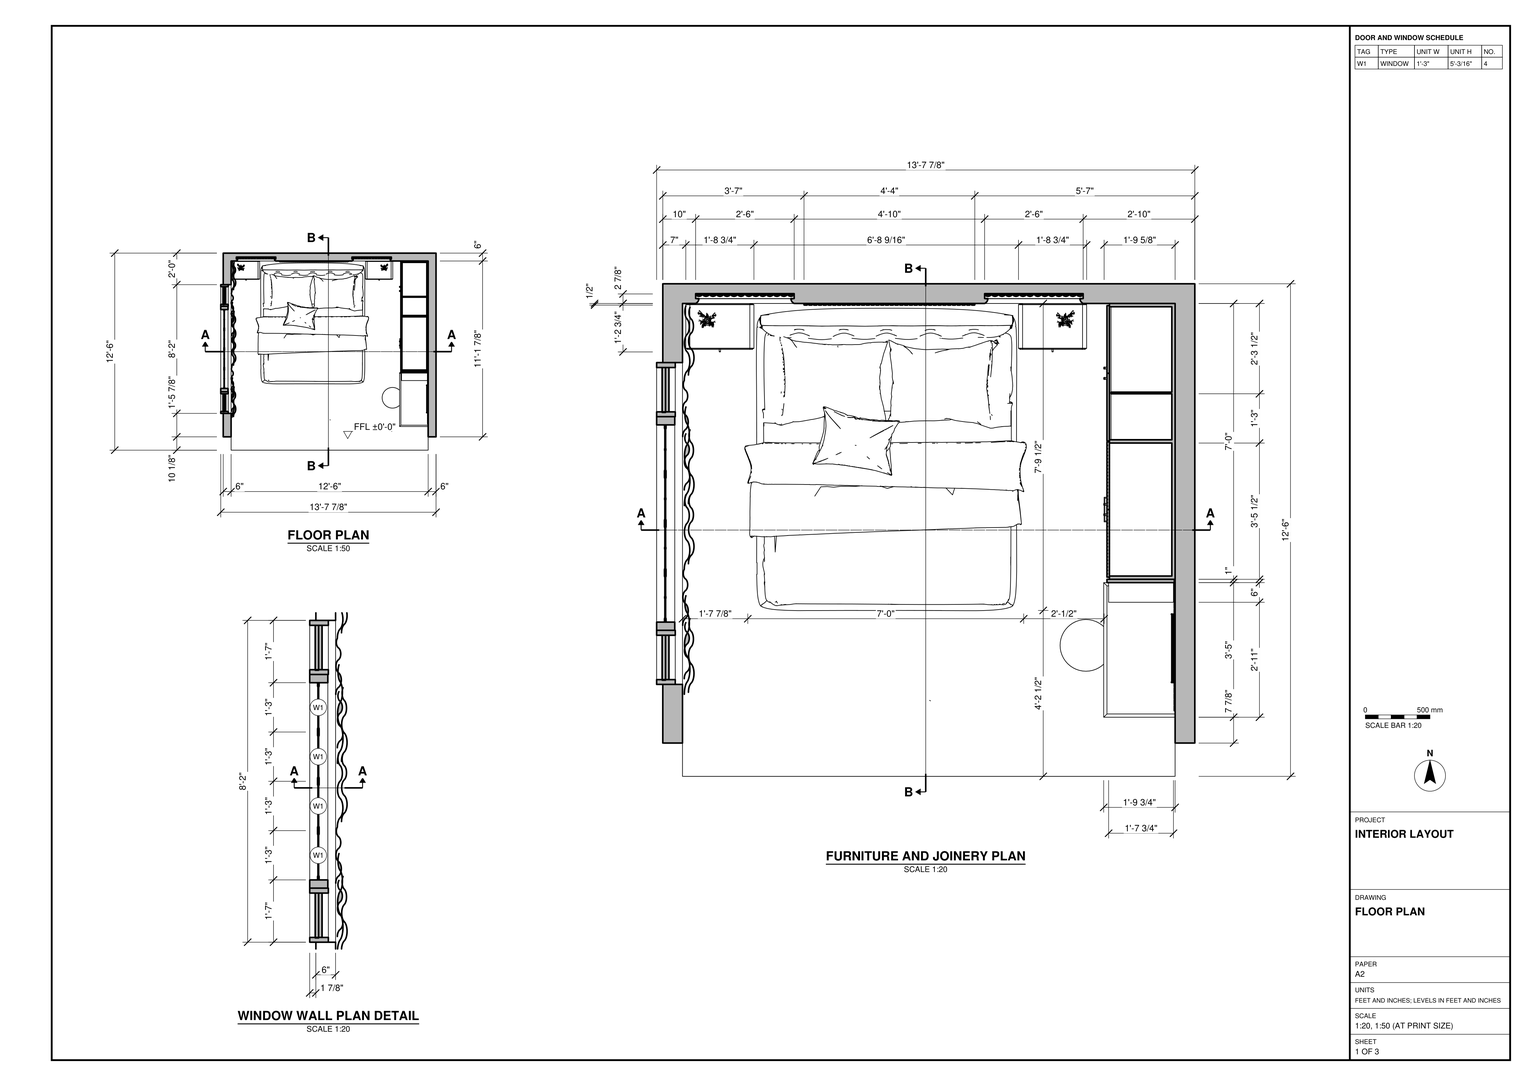
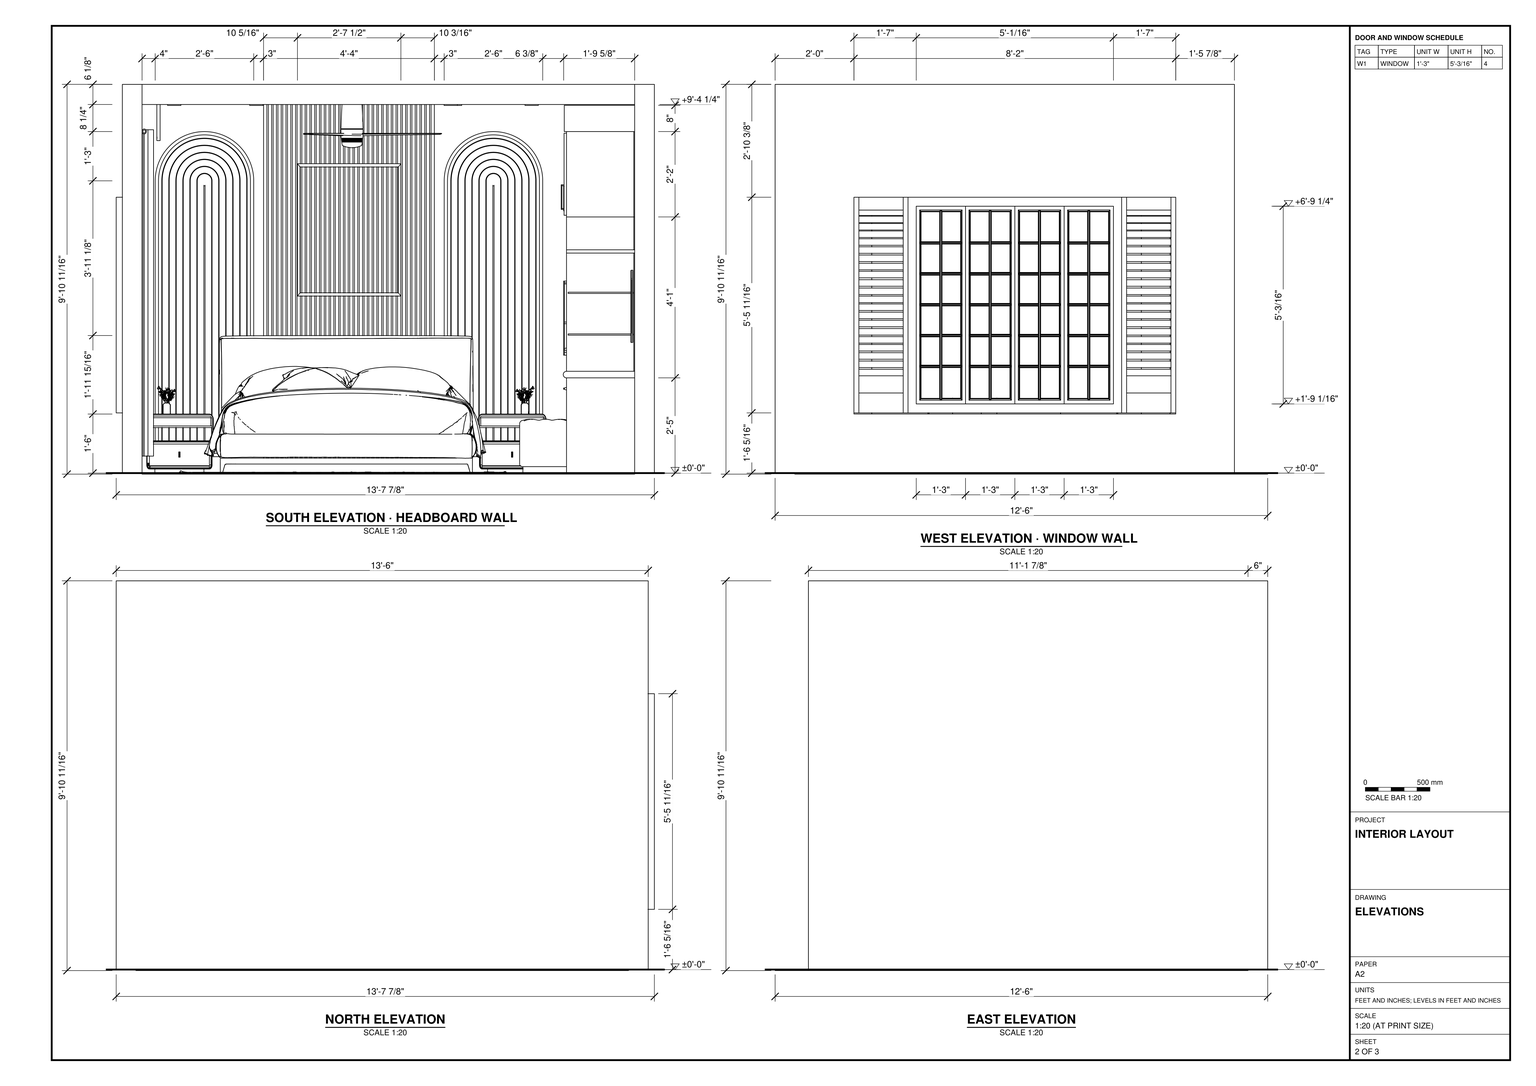
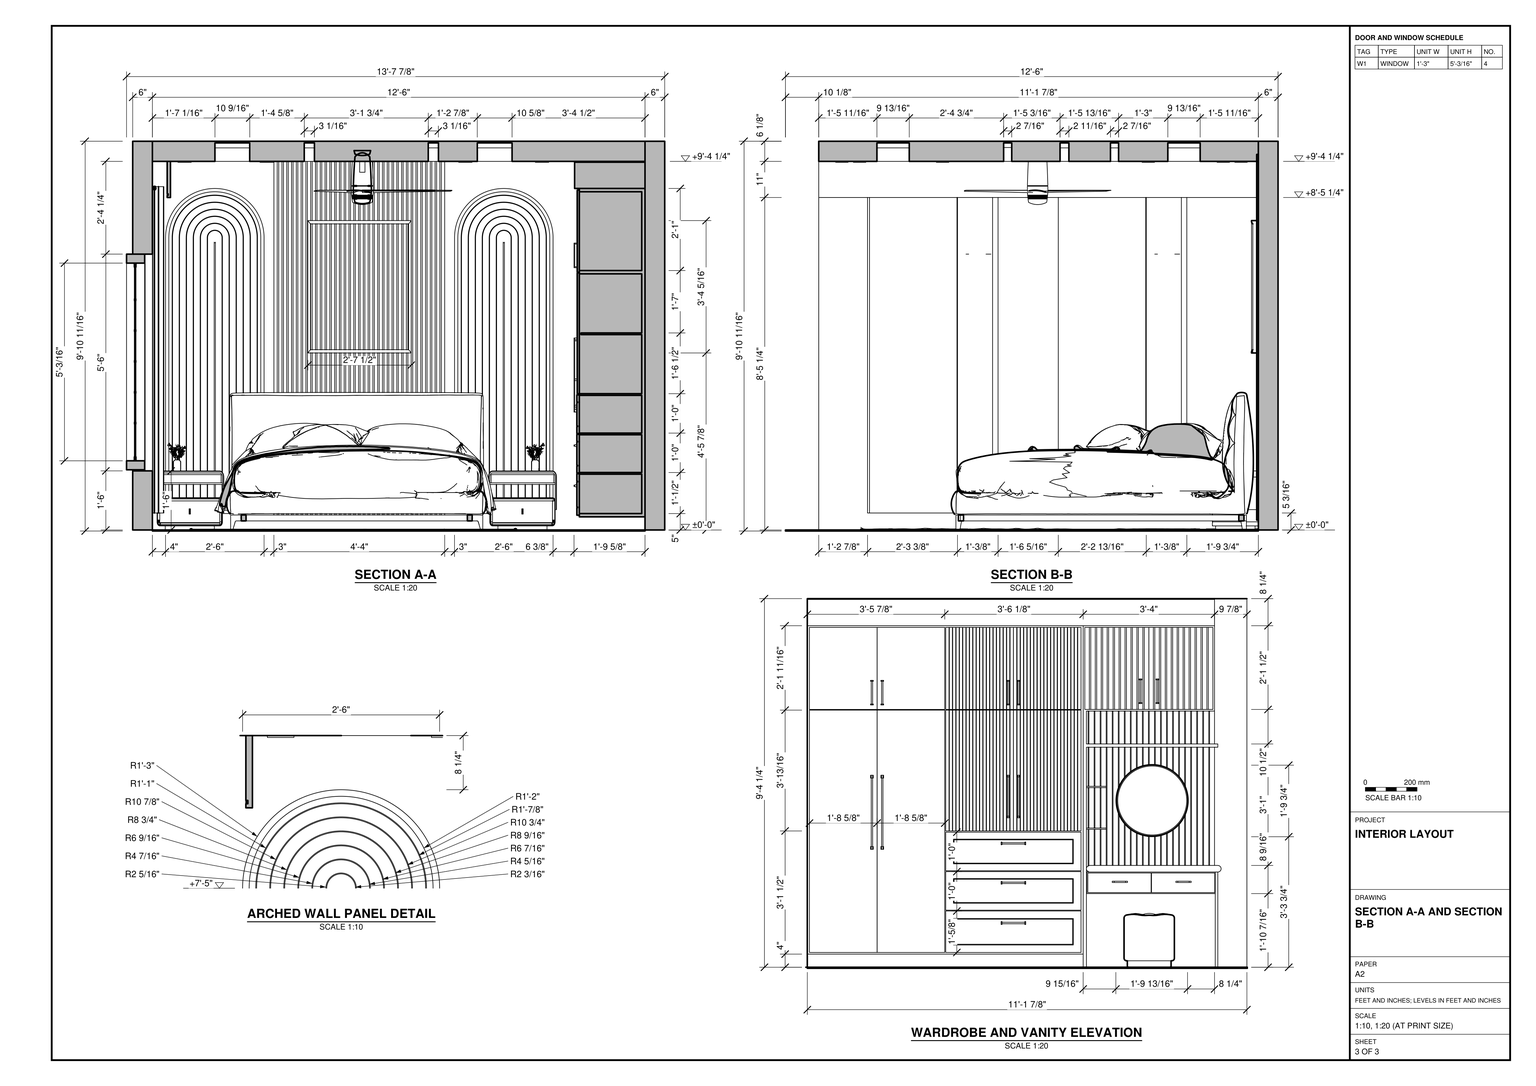
Build the furnished bedroom in SketchUp using task_files/diagram_01.pdf. Work in feet and inches. Set the finished floor at ±0'-0". The overall model is 13'-7 7/8" wide, 12'-6" deep and 9'-10 11/16" high. Model the floor, the 6" walls and the ceiling shown in section, leaving the side opposite the headboard open as drawn in plan.

Use the window wall detail to place the four glazed window units in a single framed opening, with the horizontally slatted panels at its ends and curtains on the room side. Set the bed against the headboard wall with a low bedside unit on each side. Follow the arched panel detail for the nested bands above the bedside units and the elevation for the vertically ribbed panel behind the bed. Include the framed art above the headboard and the ceiling fan over the bed.

Fit the wardrobe and vanity along the wall opposite the windows. Use the joinery elevation to distinguish the tall doors, the ribbed doors above the drawer bank, and the vanity bay with its overhead cupboard, round mirror, work surface and seat. Decor and loose items may be any suitable library components. Keep shell elements and each furniture or joinery piece in separate groups or components, and use components for repeated parts. Save one SketchUp model as output_files/bedroom_with_arched_headboard_wall_and_fitted_wardrobes.skp.

# SketchUp Ruby script. Lengths in inches.
U = 1.inch
M = Sketchup.active_model
def pt(a) = Geom::Point3d.new(a.map { |v| v * U })
def face(e, loops, mat)
  f = e.add_face(loops[0].map { |a| pt(a) })
  loops[1..].each { |l| e.add_face(l.map { |a| pt(a) }).erase! }
  f.material = f.back_material = mat if mat
  f
end
# faces: each face lists its corners as indices into pts; further lists are holes
def faces(e, pts, list, mat = nil) = list.each { |f| face(e, (f[0].is_a?(Array) ? f : [f]).map { |l| l.map { |i| pts[i] } }, mat) }
# xy, xz, yz: faces in a plane at the given z, y or x. An outline is a flat list of corners, or four numbers for a rectangle; further outlines are holes
def ring(l) = l.size == 4 ? [[l[0], l[1]], [l[2], l[1]], [l[2], l[3]], [l[0], l[3]]] : l.each_slice(2).to_a
def flat(e, list, mat, &to3) = list.each { |f| face(e, (f[0].is_a?(Array) ? f : [f]).map { |l| ring(l).map { |u, v| to3.(u, v) } }, mat) }
def xy(e, z, list, mat = nil) = flat(e, list, mat) { |x, y| [x, y, z] }
def xz(e, y, list, mat = nil) = flat(e, list, mat) { |x, z| [x, y, z] }
def yz(e, x, list, mat = nil) = flat(e, list, mat) { |y, z| [x, y, z] }
def lines(e, pts, list) = list.each { |a, b| e.add_line(pt(pts[a]), pt(pts[b])) }
# prism: a flat outline (further loops are holes) pulled along v
def prism(e, loops, v, mat = nil)
  f = face(e, loops, mat); d = Geom::Vector3d.new(v.map { |x| x * U })
  f.pushpull(f.normal.samedirection?(d) ? d.length : -d.length)
end
def box(e, o, s, mat = nil) = prism(e, [[o, [o[0] + s[0], o[1], o[2]], [o[0] + s[0], o[1] + s[1], o[2]], [o[0], o[1] + s[1], o[2]]]], [0, 0, s[2]], mat)
def at(x, y, z, deg = 0) = Geom::Transformation.translation(pt([x, y, z])) * Geom::Transformation.rotation(ORIGIN, Z_AXIS, deg.degrees)
def axes(o, x, y, z) = Geom::Transformation.new([*x, 0, *y, 0, *z, 0, *pt(o).to_a, 1])
def part(name) = M.definitions.add(name)
# library, detail: a bought-in or finely detailed component or shape, given as its bounding box
def library(name, o, s) = part(name).tap { |d| box(d.entities, o, s) }
def detail(e, o, s) = box(e.add_group.entities, o, s)
def put(e, d, t, mat = nil) = e.add_instance(d, t).tap { |i| i.material = mat if mat }
def group(e, t, mat = nil) = e.add_group.tap { |g| g.transformation = t; g.material = mat if mat }.entities
root = M.entities
M.materials.add("Carpet_Frieze_Low").color = [170, 156, 146]
M.materials.add("Carpet_Loop_Low").color = [201, 172, 127]
M.materials["Carpet_Loop_Low"].alpha = 0.3
M.materials.add("[Marble Carrara Gold Floor Tile]").color = [225, 223, 217]
c1 = part("Curtain panel")
p = [[17.625,0.0625,78.74],[17.625,0.0625,0],[18.27,0,0],[18.27,0,78.74],[18.92,0.0625,0],[18.92,0.0625,78.74],
  [17,0.25,78.74],[17,0.25,0],[19.55,0.25,0],[19.55,0.25,78.74],[16.43,0.56,78.74],[16.43,0.56,0],
  [20.12,0.56,0],[20.12,0.56,78.74],[6.31,0.6,78.74],[6.31,0.6,0],[6.8125,0.45,0],[6.8125,0.45,78.74],
  [7.33,0.4,0],[7.33,0.4,78.74],[7.86,0.45,0],[7.86,0.45,78.74],[8.36,0.6,0],[8.36,0.6,78.74],
  [5.85,0.85,78.74],[5.85,0.85,0],[8.82,0.85,0],[8.82,0.85,78.74],[15.92,0.97,78.74],[15.92,0.97,0],
  [20.625,0.97,0],[20.625,0.97,78.74],[5.44,1.18,78.74],[5.44,1.18,0],[9.23,1.18,0],[9.23,1.18,78.74],
  [15.51,1.48,78.74],[15.51,1.48,0],[21.04,1.48,0],[21.04,1.48,78.74],[5.11,1.59,78.74],[5.11,1.59,0],
  [9.5625,1.59,0],[9.5625,1.59,78.74],[14.93,2.55,78.74],[14.93,2.55,0],[15.2,2.04,0],[15.2,2.04,78.74],
  [21.34,2.04,0],[21.64,2.59,0],[21.64,2.59,78.74],[21.34,2.04,78.74],[4.63,2.47,78.74],[4.63,2.47,0],
  [4.86,2.04,0],[4.86,2.04,78.74],[9.81,2.04,0],[10.08,2.55,0],[10.08,2.55,78.74],[9.81,2.04,78.74],
  [4.32,2.85,78.74],[4.32,2.85,0],[10.44,2.99,0],[10.44,2.99,78.74],[14.57,2.99,78.74],[14.57,2.99,0],
  [22.03,3.0625,0],[22.03,3.0625,78.74],[0.85,2.85,78.74],[0.85,2.85,0],[1.22,3.15,0],[1.22,3.15,78.74],
  [3.95,3.15,78.74],[3.95,3.15,0],[10.89,3.35,0],[10.89,3.35,78.74],[14.125,3.35,78.74],[14.125,3.35,0],
  [22.5,3.45,0],[22.5,3.45,78.74],[1.65,3.375,0],[1.65,3.375,78.74],[3.53,3.375,78.74],[3.53,3.375,0],
  [2.11,3.52,0],[2.11,3.52,78.74],[3.07,3.52,78.74],[3.07,3.52,0],[11.39,3.625,0],[11.39,3.625,78.74],
  [13.62,3.625,78.74],[13.62,3.625,0],[2.59,3.5625,0],[2.59,3.5625,78.74],[23.04,3.74,0],[23.04,3.74,78.74],
  [11.9375,3.79,0],[11.9375,3.79,78.74],[13.07,3.79,78.74],[13.07,3.79,0],[23.63,3.92,0],[23.63,3.92,78.74],
  [12.51,3.85,0],[12.51,3.85,78.74],[24.25,3.98,0],[24.25,3.98,78.74],[5.51,1.25,0],[5.9,0.93,0],
  [4.95,2.09,0],[5.1875,1.64,0],[6.35,0.69,0],[6.83,0.55,0],[7.33,0.5,0],[7.84,0.55,0],
  [8.32,0.69,0],[8.77,0.93,0],[9.16,1.25,0],[9.48,1.64,0],[9.72,2.09,0],[10,2.61,0],
  [10.375,3.0625,0],[10.83,3.4375,0],[17.64,0.16,0],[18.27,0.1,0],[11.35,3.71,0],[11.92,3.89,0],
  [12.51,3.94,0],[13.09,3.89,0],[20.56,1.04,0],[20.96,1.53,0],[13.66,3.71,0],[14.18,3.4375,0],
  [14.64,3.0625,0],[15.01,2.61,0],[15.29,2.09,0],[15.59,1.53,0],[15.99,1.04,0],[16.48,0.64,0],
  [17.04,0.34,0],[18.9,0.16,0],[19.51,0.34,0],[20.07,0.64,0],[21.26,2.09,0],[21.56,2.64,0],
  [21.96,3.13,0],[22.45,3.53,0],[23,3.83,0],[23.61,4.01,0],[24.24,4.08,0]]
faces(c1.entities,p,[[0,1,2,3],[3,2,4,5],[6,7,1,0],[5,4,8,9],[10,11,7,6],[9,8,12,13],[14,15,16,17],[17,16,18,19],
  [19,18,20,21],[21,20,22,23],[24,25,15,14],[23,22,26,27],[28,29,11,10],[13,12,30,31],[32,33,25,24],[27,26,34,35],
  [36,37,29,28],[31,30,38,39],[40,41,33,32],[35,34,42,43],[44,45,46,37,36,47],[39,38,48,49,50,51],[52,53,54,41,40,55],[43,42,56,57,58,59],
  [60,61,53,52],[58,57,62,63],[64,65,45,44],[50,49,66,67],[68,69,70,71],[72,73,61,60],[63,62,74,75],[76,77,65,64],
  [67,66,78,79],[71,70,80,81],[82,83,73,72],[81,80,84,85],[86,87,83,82],[75,74,88,89],[90,91,77,76],[85,84,92,93],
  [93,92,87,86],[79,78,94,95],[89,88,96,97],[98,99,91,90],[95,94,100,101],[97,96,102,103],[103,102,99,98],[101,100,104,105]])
lines(c1.entities,p,[[106,107],[108,109],[109,106],[107,110],[110,111],[111,112],[112,113],[113,114],[114,115],[115,116],[116,117],[117,118],
  [118,119],[119,120],[120,121],[122,123],[121,124],[124,125],[125,126],[126,127],[128,129],[127,130],[130,131],[131,132],
  [132,133],[133,134],[134,135],[135,136],[136,137],[137,138],[138,122],[123,139],[139,140],[140,141],[141,128],[129,142],
  [142,143],[143,144],[144,145],[145,146],[146,147],[147,148],[148,104]])
c2 = part("Curtain rod section")
yz(c2.entities,0,[[1.55,0.61,1.31,0.64,1.08,0.73,0.88,0.88,0.73,1.08,0.64,1.31,0.61,1.55,0.64,1.79,0.73,2.02,0.88,2.22,1.08,2.37,1.31,2.46,1.55,2.49,1.79,2.46,2.02,2.37,2.22,2.22,2.37,2.02,2.46,1.79,2.49,1.55,2.46,1.31,2.37,1.08,2.22,0.88,2.02,0.73,1.79,0.64]])
yz(c2.entities,2.36,[[[1.55,0,1.15,0.05,0.78,0.21,0.45,0.45,0.21,0.78,0.05,1.15,0,1.55,0.05,1.95,0.21,2.33,0.45,2.65,0.78,2.89,1.15,3.05,1.55,3.1,1.95,3.05,2.33,2.89,2.65,2.65,2.89,2.33,3.05,1.95,3.1,1.55,3.05,1.15,2.89,0.78,2.65,0.45,2.33,0.21,1.95,0.05],[1.55,0.61,1.79,0.64,2.02,0.73,2.22,0.88,2.37,1.08,2.46,1.31,2.49,1.55,2.46,1.79,2.37,2.02,2.22,2.22,2.02,2.37,1.79,2.46,1.55,2.49,1.31,2.46,1.08,2.37,0.88,2.22,0.73,2.02,0.64,1.79,0.61,1.55,0.64,1.31,0.73,1.08,0.88,0.88,1.08,0.73,1.31,0.64]]])
yz(c2.entities,3.15,[[[1.55,0,1.95,0.05,2.33,0.21,2.65,0.45,2.89,0.78,3.05,1.15,3.1,1.55,3.05,1.95,2.89,2.33,2.65,2.65,2.33,2.89,1.95,3.05,1.55,3.1,1.15,3.05,0.78,2.89,0.45,2.65,0.21,2.33,0.05,1.95,0,1.55,0.05,1.15,0.21,0.78,0.45,0.45,0.78,0.21,1.15,0.05],[1.55,0.61,1.31,0.64,1.08,0.73,0.88,0.88,0.73,1.08,0.64,1.31,0.61,1.55,0.64,1.79,0.73,2.02,0.88,2.22,1.08,2.37,1.31,2.46,1.55,2.49,1.79,2.46,2.02,2.37,2.22,2.22,2.37,2.02,2.46,1.79,2.49,1.55,2.46,1.31,2.37,1.08,2.22,0.88,2.02,0.73,1.79,0.64]]])
yz(c2.entities,61.24,[[1.55,0.61,1.79,0.64,2.02,0.73,2.22,0.88,2.37,1.08,2.46,1.31,2.49,1.55,2.46,1.79,2.37,2.02,2.22,2.22,2.02,2.37,1.79,2.46,1.55,2.49,1.31,2.46,1.08,2.37,0.88,2.22,0.73,2.02,0.64,1.79,0.61,1.55,0.64,1.31,0.73,1.08,0.88,0.88,1.08,0.73,1.31,0.64]])
p = [[2.36,1.15,0.05],[2.36,1.55,0],[3.15,1.55,0],[3.15,1.15,0.05],[2.36,1.95,0.05],[3.15,1.95,0.05],
  [2.36,0.78,0.21],[3.15,0.78,0.21],[2.36,2.33,0.21],[3.15,2.33,0.21],[2.36,0.45,0.45],[3.15,0.45,0.45],
  [2.36,2.65,0.45],[3.15,2.65,0.45],[2.36,0.21,0.78],[3.15,0.21,0.78],[2.36,2.89,0.78],[3.15,2.89,0.78],
  [2.36,1.31,0.64],[2.36,1.08,0.73],[0,1.08,0.73],[0,1.31,0.64],[3.15,1.31,0.64],[3.15,1.08,0.73],
  [61.24,1.31,0.64],[61.24,1.08,0.73],[2.36,1.55,0.61],[0,1.55,0.61],[3.15,1.55,0.61],[61.24,1.55,0.61],
  [2.36,1.79,0.64],[0,1.79,0.64],[3.15,1.79,0.64],[61.24,1.79,0.64],[2.36,2.02,0.73],[0,2.02,0.73],
  [3.15,2.02,0.73],[61.24,2.02,0.73],[2.36,0.88,0.88],[0,0.88,0.88],[3.15,0.88,0.88],[61.24,0.88,0.88],
  [2.36,2.22,0.88],[0,2.22,0.88],[3.15,2.22,0.88],[61.24,2.22,0.88],[2.36,0.05,1.15],[3.15,0.05,1.15],
  [2.36,3.05,1.15],[3.15,3.05,1.15],[2.36,0.73,1.08],[0,0.73,1.08],[3.15,0.73,1.08],[61.24,0.73,1.08],
  [2.36,2.37,1.08],[0,2.37,1.08],[3.15,2.37,1.08],[61.24,2.37,1.08],[2.36,0,1.55],[3.15,0,1.55],
  [2.36,0.64,1.31],[0,0.64,1.31],[3.15,0.64,1.31],[61.24,0.64,1.31],[2.36,2.46,1.31],[0,2.46,1.31],
  [3.15,2.46,1.31],[61.24,2.46,1.31],[2.36,3.1,1.55],[3.15,3.1,1.55],[2.36,0.61,1.55],[0,0.61,1.55],
  [3.15,0.61,1.55],[61.24,0.61,1.55],[2.36,2.49,1.55],[0,2.49,1.55],[3.15,2.49,1.55],[61.24,2.49,1.55],
  [2.36,0.05,1.95],[3.15,0.05,1.95],[2.36,0.64,1.79],[0,0.64,1.79],[3.15,0.64,1.79],[61.24,0.64,1.79],
  [2.36,2.46,1.79],[0,2.46,1.79],[3.15,2.46,1.79],[61.24,2.46,1.79],[2.36,3.05,1.95],[3.15,3.05,1.95],
  [2.36,0.73,2.02],[0,0.73,2.02],[3.15,0.73,2.02],[61.24,0.73,2.02],[2.36,2.37,2.02],[0,2.37,2.02],
  [3.15,2.37,2.02],[61.24,2.37,2.02],[2.36,0.21,2.33],[3.15,0.21,2.33],[2.36,0.88,2.22],[0,0.88,2.22],
  [3.15,0.88,2.22],[61.24,0.88,2.22],[2.36,2.22,2.22],[0,2.22,2.22],[3.15,2.22,2.22],[61.24,2.22,2.22],
  [2.36,2.89,2.33],[3.15,2.89,2.33],[2.36,1.08,2.37],[0,1.08,2.37],[3.15,1.08,2.37],[61.24,1.08,2.37],
  [2.36,2.02,2.37],[0,2.02,2.37],[3.15,2.02,2.37],[61.24,2.02,2.37],[2.36,0.45,2.65],[3.15,0.45,2.65],
  [2.36,2.65,2.65],[3.15,2.65,2.65],[2.36,1.31,2.46],[0,1.31,2.46],[3.15,1.31,2.46],[61.24,1.31,2.46],
  [2.36,1.79,2.46],[0,1.79,2.46],[3.15,1.79,2.46],[61.24,1.79,2.46],[2.36,1.55,2.49],[0,1.55,2.49],
  [3.15,1.55,2.49],[61.24,1.55,2.49],[2.36,0.78,2.89],[3.15,0.78,2.89],[2.36,2.33,2.89],[3.15,2.33,2.89],
  [2.36,1.15,3.05],[3.15,1.15,3.05],[2.36,1.95,3.05],[3.15,1.95,3.05],[2.36,1.55,3.1],[3.15,1.55,3.1]]
faces(c2.entities,p,[[0,1,2,3],[1,4,5,2],[6,0,3,7],[4,8,9,5],[10,6,7,11],[8,12,13,9],[14,10,11,15],[12,16,17,13],
  [18,19,20,21],[19,18,22,23],[24,25,23,22],[26,18,21,27],[18,26,28,22],[29,24,22,28],[30,26,27,31],[26,30,32,28],
  [33,29,28,32],[34,30,31,35],[30,34,36,32],[37,33,32,36],[19,38,39,20],[38,19,23,40],[25,41,40,23],[42,34,35,43],
  [34,42,44,36],[45,37,36,44],[46,14,15,47],[16,48,49,17],[38,50,51,39],[50,38,40,52],[41,53,52,40],[54,42,43,55],
  [42,54,56,44],[57,45,44,56],[58,46,47,59],[50,60,61,51],[60,50,52,62],[53,63,62,52],[64,54,55,65],[54,64,66,56],
  [67,57,56,66],[48,68,69,49],[60,70,71,61],[70,60,62,72],[63,73,72,62],[74,64,65,75],[64,74,76,66],[77,67,66,76],
  [78,58,59,79],[70,80,81,71],[80,70,72,82],[73,83,82,72],[84,74,75,85],[74,84,86,76],[87,77,76,86],[68,88,89,69],
  [80,90,91,81],[90,80,82,92],[83,93,92,82],[94,84,85,95],[84,94,96,86],[97,87,86,96],[98,78,79,99],[90,100,101,91],
  [100,90,92,102],[93,103,102,92],[104,94,95,105],[94,104,106,96],[107,97,96,106],[88,108,109,89],[100,110,111,101],[110,100,102,112],
  [103,113,112,102],[114,104,105,115],[104,114,116,106],[117,107,106,116],[118,98,99,119],[108,120,121,109],[110,122,123,111],[122,110,112,124],
  [113,125,124,112],[126,114,115,127],[114,126,128,116],[129,117,116,128],[122,130,131,123],[130,122,124,132],[125,133,132,124],[130,126,127,131],
  [126,130,132,128],[133,129,128,132],[134,118,119,135],[120,136,137,121],[138,134,135,139],[136,140,141,137],[142,138,139,143],[140,142,143,141]])
c3 = part("Curtain rod assembly")
put(c3.entities,c2,axes([3.125,-0.76,-71.54],[0,0,1.25313],[0,1.25313,0],[-1.25313,0,0]))
put(c3.entities,c2,axes([3.125,3.125,81],[0,0,-1.25313],[0,-1.25313,0],[-1.25313,0,0]))
c4 = part("Group\#57")
put(c4.entities,c1,axes([-0.76,0,0],[0.8979,0,0],[0,1,0],[0,0,1]),"Carpet_Frieze_Low")
put(c4.entities,c1,axes([37.23,0,0],[0.9782,0,0],[0,1,0],[0,0,1]),"Carpet_Frieze_Low")
c5 = part("curtain2")
p = [[59.99,12.8,78.74],[59.99,12.8,-38.1875],[60.15,12.52,-38.1875],[60.15,12.52,78.74],[66.72,13.7,-38.1875],[66.72,13.7,78.74],
  [73.91,13.97,78.74],[73.91,13.97,-38.1875],[49.31,14.13,-38.1875],[49.31,14.13,78.74],[2.67,12.52,-38.1875],[2.67,12.52,78.74],
  [-8.17,14.13,-38.1875],[-8.17,14.13,78.74],[2.51,12.8,78.74],[2.51,12.8,-38.1875],[16.42,13.97,78.74],[16.42,13.97,-38.1875],
  [9.24,13.7,-38.1875],[9.24,13.7,78.74]]
lines(c5.entities,p,[[0,1],[2,3],[4,5],[6,7],[8,9],[10,11],[12,13],[14,15],[16,17],[18,19]])
put(c5.entities,c1,axes([64.94,10.15,-38.1875],[0.73,0,0],[0,1,0],[0,0,1.485]),"Carpet_Loop_Low")
put(c5.entities,c1,axes([48.6875,11.28,-38.1875],[0.73,0,0],[0,1,0],[0,0,1.485]),"Carpet_Loop_Low")
put(c5.entities,c1,axes([25.83,10.15,-38.1875],[0.96815,0,0],[0,1,0],[0,0,1.485]),"Carpet_Loop_Low")
put(c5.entities,c1,axes([56.28,10.09,-38.1875],[1.28298,0,0],[0,1,0],[0,0,1.485]),"Carpet_Loop_Low")
put(c5.entities,c3,axes([25.47,12.88,78.68],[0,0,-0.46284],[0,0.798,0],[0.798,0,0]))
put(c5.entities,c1,axes([7.46,10.15,-38.1875],[0.73,0,0],[0,1,0],[0,0,1.485]),"Carpet_Loop_Low")
put(c5.entities,c1,axes([-1.2,10.09,-38.1875],[1.28298,0,0],[0,1,0],[0,0,1.485]),"Carpet_Loop_Low")
put(c5.entities,c1,axes([-8.79,11.28,-38.1875],[0.73,0,0],[0,1,0],[0,0,1.485]),"Carpet_Loop_Low")
put(c5.entities,c1,axes([-31.65,10.15,-38.1875],[0.96815,0,0],[0,1,0],[0,0,1.485]),"Carpet_Loop_Low")
put(c5.entities,c4,axes([27.05,7.18,-38.1875],[0.98,0,0],[0,1,0],[0,0,1.485]))
put(c5.entities,c4,axes([-30.43,7.18,-38.1875],[0.98,0,0],[0,1,0],[0,0,1.485]))
c6 = part("Curtains")
put(c6.entities,c5,axes([31.62,12.15,38.1875],[1,0,0],[0,-0.79,0],[0,0,1]))
c7 = library("Group\#1",[-1.875,10.14,0],[163.875,139.86,118.375])
put(root,c6,axes([0,144,5.17],[0,-1,0],[0.54,0,0],[0,0,0.85]))
put(root,c7,at(-6,0,0))
g1 = group(root,at(0,0,0),"[Marble Carrara Gold Floor Tile]")
box(g1,[0,0,-0.3125],[150,144,0.3125])
